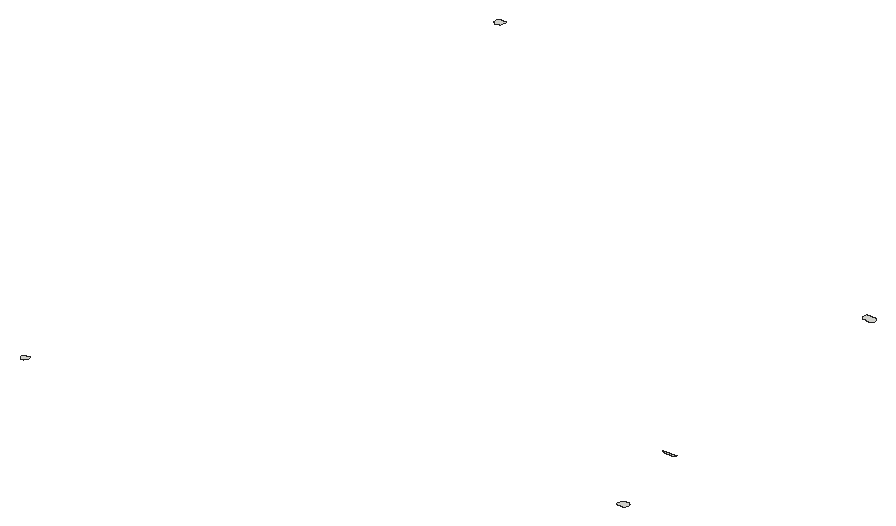
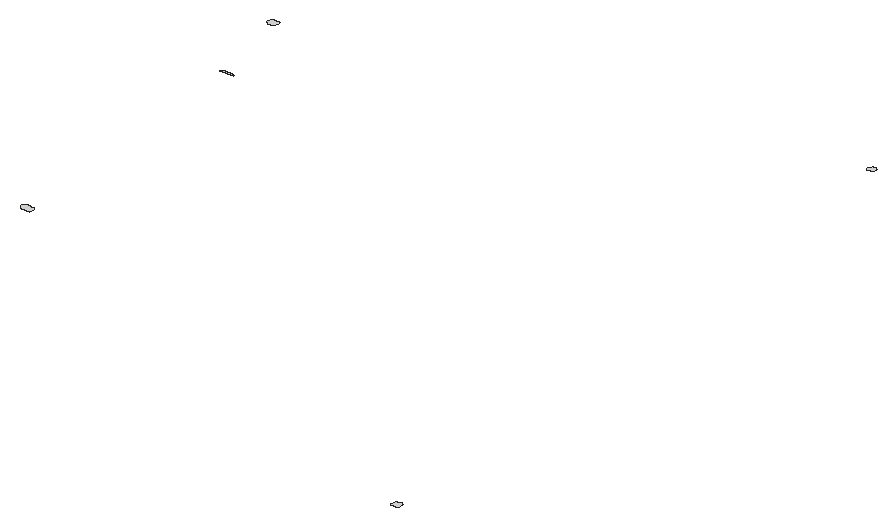
# SketchUp Ruby script. Lengths in inches.
U = 1.inch
M = Sketchup.active_model
def pt(a) = Geom::Point3d.new(a.map { |v| v * U })
def face(e, loops, mat)
  f = e.add_face(loops[0].map { |a| pt(a) })
  loops[1..].each { |l| e.add_face(l.map { |a| pt(a) }).erase! }
  f.material = f.back_material = mat if mat
  f
end
# faces: each face lists its corners as indices into pts; further lists are holes
def faces(e, pts, list, mat = nil) = list.each { |f| face(e, (f[0].is_a?(Array) ? f : [f]).map { |l| l.map { |i| pts[i] } }, mat) }
# xy, xz, yz: faces in a plane at the given z, y or x. An outline is a flat list of corners, or four numbers for a rectangle; further outlines are holes
def ring(l) = l.size == 4 ? [[l[0], l[1]], [l[2], l[1]], [l[2], l[3]], [l[0], l[3]]] : l.each_slice(2).to_a
def flat(e, list, mat, &to3) = list.each { |f| face(e, (f[0].is_a?(Array) ? f : [f]).map { |l| ring(l).map { |u, v| to3.(u, v) } }, mat) }
def xy(e, z, list, mat = nil) = flat(e, list, mat) { |x, y| [x, y, z] }
def xz(e, y, list, mat = nil) = flat(e, list, mat) { |x, z| [x, y, z] }
def yz(e, x, list, mat = nil) = flat(e, list, mat) { |y, z| [x, y, z] }
def lines(e, pts, list) = list.each { |a, b| e.add_line(pt(pts[a]), pt(pts[b])) }
# prism: a flat outline (further loops are holes) pulled along v
def prism(e, loops, v, mat = nil)
  f = face(e, loops, mat); d = Geom::Vector3d.new(v.map { |x| x * U })
  f.pushpull(f.normal.samedirection?(d) ? d.length : -d.length)
end
def box(e, o, s, mat = nil) = prism(e, [[o, [o[0] + s[0], o[1], o[2]], [o[0] + s[0], o[1] + s[1], o[2]], [o[0], o[1] + s[1], o[2]]]], [0, 0, s[2]], mat)
def at(x, y, z, deg = 0) = Geom::Transformation.translation(pt([x, y, z])) * Geom::Transformation.rotation(ORIGIN, Z_AXIS, deg.degrees)
def axes(o, x, y, z) = Geom::Transformation.new([*x, 0, *y, 0, *z, 0, *pt(o).to_a, 1])
def part(name) = M.definitions.add(name)
# library, detail: a bought-in or finely detailed component or shape, given as its bounding box
def library(name, o, s) = part(name).tap { |d| box(d.entities, o, s) }
def detail(e, o, s) = box(e.add_group.entities, o, s)
def put(e, d, t, mat = nil) = e.add_instance(d, t).tap { |i| i.material = mat if mat }
def group(e, t, mat = nil) = e.add_group.tap { |g| g.transformation = t; g.material = mat if mat }.entities
root = M.entities
xy(root,0,[[5.842,357.842,5.869,357.842,5.882,357.844,5.895,357.847,5.903,357.849,5.906,357.851,5.91,357.853,5.916,357.857,5.919,357.86,5.922,357.862,5.924,357.864,5.925,357.866,5.927,357.868,5.931,357.876,5.931,357.878,5.932,357.88,5.932,357.892,5.931,357.895,5.93,357.899,5.927,357.908,5.907,357.938,5.887,357.961,5.878,357.969,5.868,357.977,5.867,357.978,5.866,357.978,5.864,357.979,5.863,357.98,5.86,357.98,5.858,357.981,5.852,357.981,5.851,357.98,5.848,357.98,5.846,357.979,5.845,357.978,5.844,357.978,5.842,357.977,5.824,357.961,5.804,357.938,5.784,357.908,5.783,357.905,5.781,357.902,5.78,357.899,5.779,357.895,5.779,357.88,5.78,357.878,5.78,357.876,5.785,357.866,5.787,357.864,5.788,357.862,5.791,357.86,5.794,357.857,5.798,357.855,5.804,357.851,5.808,357.849,5.812,357.848,5.815,357.847,5.829,357.844],[15.247,359.86,15.261,359.861,15.289,359.865,15.298,359.868,15.316,359.876,15.324,359.881,15.329,359.884,15.334,359.889,15.339,359.893,15.347,359.903,15.351,359.909,15.352,359.911,15.355,359.92,15.355,359.924,15.356,359.927,15.356,359.935,15.355,359.941,15.353,359.951,15.349,359.961,15.343,359.971,15.337,359.979,15.333,359.982,15.327,359.988,15.311,359.996,15.299,359.999,15.279,359.999,15.273,359.998,15.268,359.996,15.262,359.994,15.251,359.99,15.241,359.985,15.231,359.979,15.221,359.972,15.212,359.965,15.195,359.948,15.188,359.939,15.18,359.927,15.179,359.924,15.177,359.92,15.175,359.914,15.175,359.91,15.174,359.907,15.174,359.901,15.175,359.899,15.175,359.894,15.18,359.884,15.186,359.878,15.189,359.876,15.192,359.873,15.198,359.869,15.202,359.868,15.205,359.866,15.209,359.865,15.218,359.863,15.228,359.861,15.238,359.861],[14.869,361.469,14.935,361.473,14.963,361.477,14.99,361.483,14.993,361.483,14.999,361.486,15.001,361.488,15.003,361.489,15.005,361.491,15.007,361.492,15.008,361.494,15.009,361.495,15.01,361.497,15.01,361.501,15.006,361.505,15.005,361.505,14.989,361.509,14.972,361.511,14.956,361.513,14.869,361.514,14.781,361.513,14.765,361.511,14.748,361.509,14.732,361.505,14.731,361.505,14.728,361.502,14.728,361.501,14.727,361.499,14.727,361.498,14.728,361.497,14.728,361.495,14.729,361.494,14.73,361.492,14.732,361.491,14.734,361.489,14.736,361.488,14.738,361.486,14.744,361.483,14.747,361.483,14.774,361.477,14.802,361.473],[14.664,366.333,14.69,366.334,14.716,366.338,14.722,366.339,14.729,366.341,14.747,366.35,14.752,366.353,14.755,366.355,14.761,366.361,14.762,366.363,14.764,366.366,14.765,366.368,14.767,366.374,14.768,366.376,14.769,366.379,14.769,366.39,14.768,366.392,14.768,366.394,14.767,366.396,14.766,366.399,14.764,366.403,14.76,366.409,14.756,366.414,14.751,366.42,14.746,366.425,14.74,366.429,14.729,366.4375,14.717,366.445,14.704,366.452,14.691,366.458,14.677,366.463,14.662,366.467,14.649,366.47,14.635,366.472,14.611,366.472,14.602,366.471,14.592,366.469,14.583,366.467,14.576,366.465,14.569,366.462,14.556,366.456,14.55,366.452,14.546,366.449,14.542,366.445,14.538,366.442,14.535,366.4375,14.531,366.433,14.528,366.429,14.527,366.426,14.525,366.423,14.524,366.42,14.523,366.416,14.521,366.41,14.521,366.395,14.523,366.389,14.525,366.385,14.526,366.382,14.53,366.378,14.531,366.376,14.549,366.361,14.556,366.357,14.5625,366.353,14.574,366.348,14.585,366.344,14.609,366.338,14.636,366.334],[5.006,369.813,5.016,369.813,5.044,369.815,5.058,369.818,5.076,369.824,5.084,369.829,5.093,369.833,5.103,369.841,5.108,369.846,5.116,369.856,5.118,369.859,5.119,369.861,5.121,369.864,5.124,369.873,5.124,369.879,5.125,369.883,5.124,369.888,5.124,369.893,5.123,369.899,5.121,369.904,5.12,369.909,5.117,369.914,5.115,369.919,5.112,369.923,5.109,369.928,5.099,369.938,5.095,369.94,5.092,369.943,5.084,369.947,5.08,369.948,5.076,369.95,5.068,369.952,5.053,369.952,5.048,369.951,5.036,369.949,5.031,369.947,5.02,369.943,5,369.932,4.99,369.925,4.972,369.909,4.964,369.901,4.957,369.892,4.949,369.88,4.947,369.876,4.944,369.867,4.944,369.863,4.943,369.86,4.943,369.852,4.944,369.849,4.944,369.847,4.949,369.837,4.951,369.835,4.952,369.833,4.955,369.831,4.958,369.828,4.967,369.822,4.971,369.821,4.974,369.819,4.978,369.818,4.987,369.816,4.997,369.814]])
